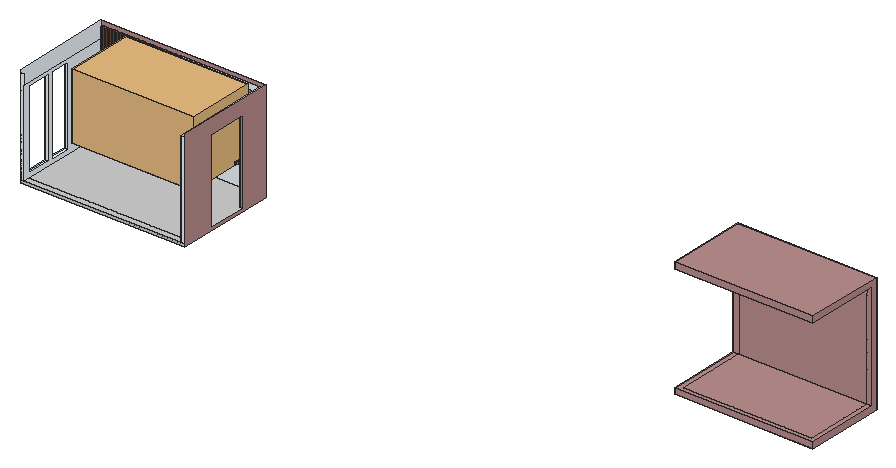
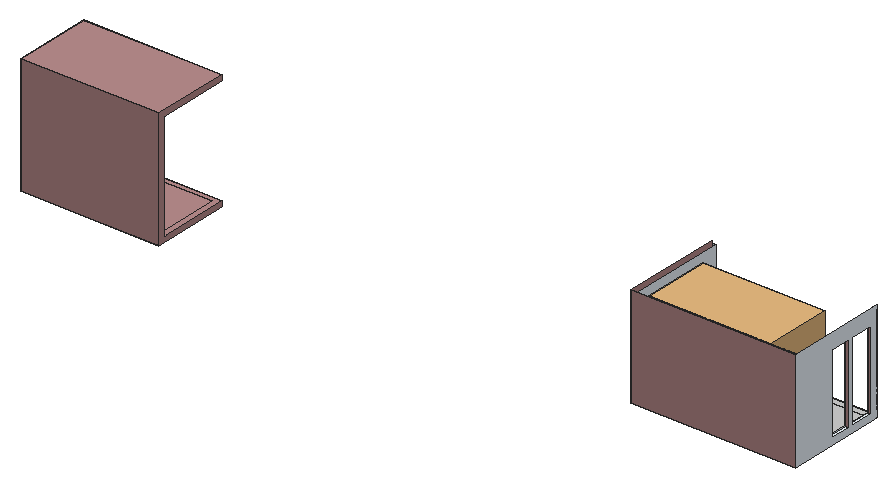
# SketchUp Ruby script. Lengths in inches.
U = 1.inch
M = Sketchup.active_model
def pt(a) = Geom::Point3d.new(a.map { |v| v * U })
def face(e, loops, mat)
  f = e.add_face(loops[0].map { |a| pt(a) })
  loops[1..].each { |l| e.add_face(l.map { |a| pt(a) }).erase! }
  f.material = f.back_material = mat if mat
  f
end
# faces: each face lists its corners as indices into pts; further lists are holes
def faces(e, pts, list, mat = nil) = list.each { |f| face(e, (f[0].is_a?(Array) ? f : [f]).map { |l| l.map { |i| pts[i] } }, mat) }
# xy, xz, yz: faces in a plane at the given z, y or x. An outline is a flat list of corners, or four numbers for a rectangle; further outlines are holes
def ring(l) = l.size == 4 ? [[l[0], l[1]], [l[2], l[1]], [l[2], l[3]], [l[0], l[3]]] : l.each_slice(2).to_a
def flat(e, list, mat, &to3) = list.each { |f| face(e, (f[0].is_a?(Array) ? f : [f]).map { |l| ring(l).map { |u, v| to3.(u, v) } }, mat) }
def xy(e, z, list, mat = nil) = flat(e, list, mat) { |x, y| [x, y, z] }
def xz(e, y, list, mat = nil) = flat(e, list, mat) { |x, z| [x, y, z] }
def yz(e, x, list, mat = nil) = flat(e, list, mat) { |y, z| [x, y, z] }
def lines(e, pts, list) = list.each { |a, b| e.add_line(pt(pts[a]), pt(pts[b])) }
# prism: a flat outline (further loops are holes) pulled along v
def prism(e, loops, v, mat = nil)
  f = face(e, loops, mat); d = Geom::Vector3d.new(v.map { |x| x * U })
  f.pushpull(f.normal.samedirection?(d) ? d.length : -d.length)
end
def box(e, o, s, mat = nil) = prism(e, [[o, [o[0] + s[0], o[1], o[2]], [o[0] + s[0], o[1] + s[1], o[2]], [o[0], o[1] + s[1], o[2]]]], [0, 0, s[2]], mat)
def at(x, y, z, deg = 0) = Geom::Transformation.translation(pt([x, y, z])) * Geom::Transformation.rotation(ORIGIN, Z_AXIS, deg.degrees)
def axes(o, x, y, z) = Geom::Transformation.new([*x, 0, *y, 0, *z, 0, *pt(o).to_a, 1])
def part(name) = M.definitions.add(name)
# library, detail: a bought-in or finely detailed component or shape, given as its bounding box
def library(name, o, s) = part(name).tap { |d| box(d.entities, o, s) }
def detail(e, o, s) = box(e.add_group.entities, o, s)
def put(e, d, t, mat = nil) = e.add_instance(d, t).tap { |i| i.material = mat if mat }
def group(e, t, mat = nil) = e.add_group.tap { |g| g.transformation = t; g.material = mat if mat }.entities
root = M.entities
M.materials.add("[0093_AliceBlue]").color = [240, 248, 255]
M.materials.add("[0095_LightBlue]").color = [173, 216, 230]
M.materials.add("[0119_RosyBrown]").color = [188, 143, 143]
M.materials.add("[Carrera Marble]").color = [207, 207, 207]
M.materials.add("[Sandstone]").color = [118, 81, 52]
c1 = library("Group\#4",[-0.5,-0.5,0],[110.4375,24.3125,2.25])
c2 = library("Group\#2",[-0.5,-0.5,0],[66.38,2.78,72.7])
c3 = library("Group\#3",[-0.5,-0.5,0],[27.47,2.78,72.7])
c4 = library("Group\#5",[-0.5,-0.5,0],[170.54,94.85,92.14])
xy(root,0,[[0,0,230.5,141.75]],"[0093_AliceBlue]")
xy(root,0,[[853.51,78.57,1047.76,189.2]],"[0119_RosyBrown]")
xy(root,3.9375,[[4.95,112.24,14.18,112.24,12.9,112.62,11.89,113.04,11.67,113.13,10.5,113.79,9.83,114.27,9.42,114.56,8.43,115.46,7.54,116.46,7.01,117.21,6.77,117.55,6.125,118.72,5.61,119.96,5.25,121.24,5.02,122.56,4.95,123.89],[14.18,112.24,14.71,112.24,14.71,135.55,11.89,135.55,11.89,113.04,12.9,112.62],[14.71,112.24,16.77,137.93],[16.77,112.24,19.59,137.93],[19.59,112.24,21.65,137.93],
  [21.65,112.24,24.47,137.93],[24.47,112.24,26.53,135.55],[26.53,112.24,29.35,137.93],[29.35,112.24,31.42,137.93],[31.42,112.24,34.23,137.93],
  [34.23,112.24,36.3,137.93],[36.3,112.24,39.11,137.93],[39.11,112.24,41.18,137.93],[41.18,112.24,43.99,137.93],[43.99,112.24,46.06,137.93],
  [46.06,112.24,48.875,137.93],[48.875,112.24,50.9375,137.93],[50.9375,112.24,53.76,137.93],[53.76,112.24,55.82,137.93],[55.82,112.24,58.64,137.93],
  [58.64,112.24,60.7,137.93],[60.7,112.24,63.52,137.93],[63.52,112.24,65.58,137.93],[65.58,112.24,68.4,137.93],[68.4,112.24,70.46,137.93],
  [70.46,112.24,73.28,137.93],[73.28,112.24,75.34,137.93],[75.34,112.24,78.16,137.93],[78.16,112.24,80.22,137.93],[80.22,112.24,83.04,137.93],
  [83.04,112.24,85.1,137.93],[85.1,112.24,87.92,137.93],[87.92,112.24,89.98,137.93],[89.98,112.24,92.8,137.93],[92.8,112.24,94.86,137.93],
  [94.86,112.24,97.68,137.93],[97.68,112.24,99.74,137.93],[99.74,112.24,102.5625,137.93],[102.5625,112.24,103.53,112.24,104.625,112.3125,104.625,135.55,102.5625,135.55],[104.625,112.3125,105.02,112.34,106.47,112.64,107.44,112.99,107.44,135.55,104.625,135.55],
  [107.44,112.99,107.875,113.14,109.2,113.83,109.51,114.05,109.51,135.55,107.44,135.55],[11.89,113.04,11.89,135.55,9.83,135.55,9.83,114.27,10.5,113.79,11.67,113.13],[109.51,114.05,110.41,114.6875,111.5,115.7,112.32,116.72,112.32,135.55,109.51,135.55],[9.83,114.27,9.83,135.55,7.01,135.55,7.01,117.21,7.54,116.46,8.43,115.46,9.42,114.56],[112.32,116.72,112.43,116.86,113.2,118.13,113.79,119.5,114.05,120.42,114.05,135.55,112.32,135.55],
  [114.05,120.42,114.19,120.93,114.39,122.375,114.39,135.55,114.05,135.55],[7.01,135.55,9.83,137.93],[9.83,135.55,11.89,137.93],[11.89,135.55,14.71,137.93],[24.47,135.55,26.53,137.93],
  [102.5625,135.55,104.625,137.93],[104.625,135.55,107.44,137.93],[107.44,135.55,109.51,137.93],[109.51,135.55,112.32,137.93],[112.32,135.55,114.05,137.93],
  [114.05,135.55,114.39,137.93]],"[0119_RosyBrown]")
xy(root,3.9375,[[4.95,0,225.375,9.26],[4.95,9.26,225.375,9.26,225.375,45.11,230.5,45.11,230.5,101.93,225.375,101.93,225.375,137.93,114.39,137.93,114.39,122.375,114.19,120.93,114.05,120.42,113.79,119.5,113.2,118.13,112.43,116.86,112.32,116.72,111.5,115.7,110.41,114.6875,109.51,114.05,109.2,113.83,107.875,113.14,107.44,112.99,106.47,112.64,105.02,112.34,104.625,112.3125,103.53,112.24,4.95,112.24]],"[Carrera Marble]")
xy(root,7.75,[[853.51,78.57,1047.76,78.57,1047.76,181.57,1040.13,181.57,1040.13,86.2,861.13,86.2,861.13,181.57,853.51,181.57],[861.13,86.2,1040.13,181.57]],"[0119_RosyBrown]")
xy(root,9.5,[[0,9.26,4.95,43.72],[0,48.29,4.95,77.05]],"[0093_AliceBlue]")
xy(root,9.5,[[0,43.72,4.95,48.29]],"[0119_RosyBrown]")
xy(root,15.0625,[[14.18,112.24,103.53,115.3]],"[0119_RosyBrown]")
xy(root,16.4375,[[14.18,112.24,103.53,115.3]],"[0119_RosyBrown]")
xy(root,30.75,[[14.18,112.24,103.53,112.24,105.02,112.34,106.47,112.64,107.875,113.14,109.2,113.83,110.41,114.6875,111.5,115.7,112.43,116.86,113.2,118.13,113.79,119.5,114.19,120.93,114.39,122.375,114.39,135.55,4.95,135.55,4.95,123.89,5.02,122.56,5.25,121.24,5.61,119.96,6.125,118.72,6.77,117.55,7.54,116.46,8.43,115.46,9.42,114.56,10.5,113.79,11.67,113.13,12.9,112.62]],"[0119_RosyBrown]")
xy(root,35.24,[[4.97,133.77,70.35,135.55],[87.92,133.77,114.39,135.55]],"[0095_LightBlue]")
xy(root,46.22,[[[137.0625,109.13,135.97,109.21,135.02,109.41,134.1,109.73,133.23,110.18,132.43,110.74,131.72,111.4,131.1,112.16,130.59,112.99,130.2,113.88,129.93,114.82,129.79,115.78,129.78,116.98,129.78,134.53,209.98,134.53,209.98,117.22,209.81,116.2,209.49,115.13,209.04,114.11,208.48,113.15,207.8,112.27,207.02,111.48,206.15,110.79,205.2,110.21,204.18,109.74,203.125,109.41,202.03,109.21,200.8125,109.13],[137.09,109.92,200.79,109.92,201.93,109.99,202.93,110.18,203.9,110.48,204.83,110.9,205.69,111.43,206.49,112.07,207.2,112.79,207.82,113.6,208.34,114.47,208.75,115.4,209.04,116.38,209.19,117.29,209.19,133.74,130.57,133.74,130.57,116.98,130.58,115.84,130.7,114.98,130.94,114.15,131.29,113.35,131.74,112.61,132.29,111.94,132.93,111.35,133.64,110.85,134.41,110.46,135.23,110.17,136.08,109.99]]],"[0119_RosyBrown]")
xy(root,47.91,[[[136.95,105.74,135.51,105.84,134.1,106.13,132.75,106.61,131.47,107.27,130.29,108.09,129.24,109.07,128.33,110.18,127.57,111.41,127,112.72,126.6,114.11,126.4,115.53,126.39,116.97,126.39,137.93,213.375,137.93,213.375,116.94,213.12,115.43,212.68,113.96,212.07,112.5625,211.3,111.25,210.36,110.04,209.29,108.95,208.1,108,206.79,107.2,205.4,106.57,203.95,106.11,202.44,105.83,200.92,105.74],[137.0625,109.13,200.8125,109.13,202.03,109.21,203.125,109.41,204.18,109.74,205.2,110.21,206.15,110.79,207.02,111.48,207.8,112.27,208.48,113.15,209.04,114.11,209.49,115.13,209.81,116.2,209.98,117.22,209.98,134.53,129.78,134.53,129.78,116.98,129.79,115.78,129.93,114.82,130.2,113.88,130.59,112.99,131.1,112.16,131.72,111.4,132.43,110.74,133.23,110.18,134.1,109.73,135.02,109.41,135.97,109.21]],[137.09,109.92,136.08,109.99,135.23,110.17,134.41,110.46,133.64,110.85,132.93,111.35,132.29,111.94,131.74,112.61,131.29,113.35,130.94,114.15,130.7,114.98,130.58,115.84,130.57,116.98,130.57,133.74,209.19,133.74,209.19,117.29,209.04,116.38,208.75,115.4,208.34,114.47,207.82,113.6,207.2,112.79,206.49,112.07,205.69,111.43,204.83,110.9,203.9,110.48,202.93,110.18,201.93,109.99,200.79,109.92]],"[0119_RosyBrown]")
xy(root,51.66,[[136.95,105.74,200.92,105.74,202.44,105.83,203.95,106.11,205.4,106.57,206.79,107.2,208.1,108,209.29,108.95,210.36,110.04,211.3,111.25,212.07,112.5625,212.68,113.96,213.12,115.43,213.375,116.94,213.375,137.93,126.39,137.93,126.39,116.97,126.4,115.53,126.6,114.11,127,112.72,127.57,111.41,128.33,110.18,129.24,109.07,130.29,108.09,131.47,107.27,132.75,106.61,134.1,106.13,135.51,105.84]],"[0119_RosyBrown]")
xy(root,107.93,[[101.15,133.77,114.39,135.55]],"[0095_LightBlue]")
xy(root,157.52,[[853.51,78.57,861.13,181.57],[861.13,78.57,1040.13,181.57],[1040.13,78.57,1047.76,181.57]],"[0119_RosyBrown]")
xy(root,166,[[853.51,78.57,1047.76,189.2]],"[0119_RosyBrown]")
xz(root,0,[[0,3.9375,4.95,138.36],[225.375,3.9375,230.5,138.36]],"[0093_AliceBlue]")
xz(root,0,[[0,0,230.5,3.9375]],"[Carrera Marble]")
xz(root,9.26,[[0,9.5,4.95,119.86]],"[0119_RosyBrown]")
xz(root,43.72,[[0,9.5,4.95,119.86]],"[0093_AliceBlue]")
xz(root,45.11,[[225.375,3.9375,230.5,121.64]],"[0119_RosyBrown]")
xz(root,48.29,[[0,9.5,4.95,119.86]],"[0119_RosyBrown]")
xz(root,77.05,[[0,9.5,4.95,119.86]],"[0093_AliceBlue]")
xz(root,78.57,[[853.51,0,1047.76,7.75],[853.51,157.52,1047.76,166]],"[0119_RosyBrown]")
xz(root,101.93,[[225.375,3.9375,230.5,121.64]],"[0119_RosyBrown]")
xz(root,105.74,[[136.95,47.91,200.92,51.66]],"[0119_RosyBrown]")
xz(root,109.13,[[137.0625,46.22,200.8125,46.6],[137.0625,46.6,200.8125,47.91]],"[0119_RosyBrown]")
xz(root,109.92,[[137.09,46.22,200.79,46.6],[137.09,46.6,200.79,47.91]],"[0119_RosyBrown]")
xz(root,112.24,[[14.18,3.9375,103.53,15.0625],[14.18,16.4375,103.53,28.5]],"[0119_RosyBrown]")
xz(root,115.3,[[14.18,15.0625,103.53,16.4375]],"[0119_RosyBrown]")
xz(root,131.99,[[4.97,35.24,70.35,35.24,70.35,92.61,70.01,94.53,69.47,96.4,68.71,98.19,67.77,99.89,66.64,101.48,65.34,102.93,63.89,104.22,62.31,105.35,60.61,106.3,58.8125,107.05,56.95,107.6,55.03,107.93,4.97,107.93],[87.92,35.24,114.39,35.24,114.39,107.93,101.15,107.93,99.43,107.82,97.73,107.48,96.09,106.93,94.54,106.16,93.1,105.2,91.8,104.06,90.66,102.76,89.69,101.32,88.93,99.76,88.37,98.125,88.03,96.43,87.92,94.7]],"[0095_LightBlue]")
xz(root,133.74,[[130.57,46.22,209.19,46.6],[130.57,46.6,209.19,47.91]],"[0119_RosyBrown]")
xz(root,134.53,[[129.78,46.22,209.98,46.6],[129.78,46.6,209.98,47.91]],"[0119_RosyBrown]")
xz(root,135.55,[[4.95,3.9375,26.53,30.75],[26.53,3.9375,114.39,30.75],[4.95,35.24,4.97,107.93],[4.97,35.24,26.53,107.93],[26.53,35.24,26.53,107.93,55.03,107.93,56.95,107.6,58.8125,107.05,60.61,106.3,62.31,105.35,63.89,104.22,65.34,102.93,66.64,101.48,67.77,99.89,68.71,98.19,69.47,96.4,70.01,94.53,70.35,92.61,70.35,35.24],
  [87.92,35.24,87.92,94.7,88.03,96.43,88.37,98.125,88.93,99.76,89.69,101.32,90.66,102.76,91.8,104.06,93.1,105.2,94.54,106.16,96.09,106.93,97.73,107.48,99.43,107.82,101.15,107.93,114.39,107.93,114.39,35.24]],"[0119_RosyBrown]")
xz(root,137.93,[[7.01,3.9375,9.83,138.36],[11.89,3.9375,14.71,138.36],[16.77,3.9375,19.59,138.36],[21.65,3.9375,24.47,138.36],[26.53,3.9375,29.35,138.36],
  [31.42,3.9375,34.23,138.36],[36.3,3.9375,39.11,138.36],[41.18,3.9375,43.99,138.36],[46.06,3.9375,48.875,138.36],[50.9375,3.9375,53.76,138.36],
  [55.82,3.9375,58.64,138.36],[60.7,3.9375,63.52,138.36],[65.58,3.9375,68.4,138.36],[70.46,3.9375,73.28,138.36],[75.34,3.9375,78.16,138.36],
  [80.22,3.9375,83.04,138.36],[85.1,3.9375,87.92,138.36],[89.98,3.9375,92.8,138.36],[94.86,3.9375,97.68,138.36],[99.74,3.9375,102.5625,138.36],
  [104.625,3.9375,107.44,138.36],[109.51,3.9375,112.32,138.36],[[114.39,3.9375,225.375,138.36],[189.375,103.42,213.375,130.36],[151.09,86.86,188.68,103.11],[151.09,115.49,188.68,130.36],[151.09,103.42,188.68,115.3],[189.375,86.86,213.375,103.11],[126.39,86.86,150.39,102.8],[126.39,115.49,150.39,130.36],[126.39,47.91,213.375,51.66],[126.39,103.42,150.39,115.3]]],"[0093_AliceBlue]")
xz(root,137.93,[[9.83,3.9375,11.89,138.36],[14.71,3.9375,16.77,138.36],[19.59,3.9375,21.65,138.36],[24.47,3.9375,26.53,138.36],[29.35,3.9375,31.42,138.36],
  [34.23,3.9375,36.3,138.36],[39.11,3.9375,41.18,138.36],[43.99,3.9375,46.06,138.36],[48.875,3.9375,50.9375,138.36],[53.76,3.9375,55.82,138.36],
  [58.64,3.9375,60.7,138.36],[63.52,3.9375,65.58,138.36],[68.4,3.9375,70.46,138.36],[73.28,3.9375,75.34,138.36],[78.16,3.9375,80.22,138.36],
  [83.04,3.9375,85.1,138.36],[87.92,3.9375,89.98,138.36],[92.8,3.9375,94.86,138.36],[97.68,3.9375,99.74,138.36],[102.5625,3.9375,104.625,138.36],
  [107.44,3.9375,109.51,138.36],[112.32,3.9375,114.05,138.36],[114.05,3.9375,114.39,138.36]],"[0119_RosyBrown]")
xz(root,141.75,[[0,0,230.5,141.75]],"[0119_RosyBrown]")
xz(root,181.57,[[853.51,7.75,861.13,157.52],[861.13,7.75,1040.13,157.52],[1040.13,7.75,1047.76,157.52]],"[0119_RosyBrown]")
xz(root,189.2,[[853.51,0,1047.76,166]],"[0119_RosyBrown]")
yz(root,0,[[[0,0,141.75,141.75],[9.26,9.5,43.72,9.5,43.72,119.86,48.29,119.86,48.29,9.5,77.05,9.5,77.05,119.86,9.26,119.86]]],"[0093_AliceBlue]")
yz(root,4.95,[[[0,3.9375,123.89,3.9375,123.89,30.75,135.55,30.75,135.55,3.9375,137.93,3.9375,137.93,138.36,135.55,138.36,135.55,123.05,0,123.05],[9.26,9.5,9.26,119.86,77.05,119.86,77.05,9.5,48.29,9.5,48.29,119.86,43.72,119.86,43.72,9.5]]],"[0093_AliceBlue]")
yz(root,4.95,[[123.89,3.9375,135.55,28.5],[123.89,28.5,135.55,30.75]],"[0119_RosyBrown]")
yz(root,4.97,[[131.99,35.24,133.77,107.93],[133.77,35.24,135.55,107.93]],"[0119_RosyBrown]")
yz(root,14.18,[[112.24,15.0625,115.3,16.4375]],"[0119_RosyBrown]")
yz(root,26.53,[[135.55,3.9375,137.93,138.36]],"[Sandstone]")
yz(root,70.35,[[133.77,35.24,135.55,92.61]],"[0095_LightBlue]")
yz(root,87.92,[[133.77,35.24,135.55,94.7]],"[0119_RosyBrown]")
yz(root,103.53,[[112.24,15.0625,115.3,16.4375]],"[0119_RosyBrown]")
yz(root,114.39,[[133.77,35.24,135.55,107.93]],"[0095_LightBlue]")
yz(root,114.39,[[122.375,3.9375,135.55,28.5]],"[0119_RosyBrown]")
yz(root,126.39,[[116.97,47.91,137.93,51.66]],"[0119_RosyBrown]")
yz(root,129.78,[[116.98,46.22,134.53,46.6],[116.98,46.6,134.53,47.91]],"[0119_RosyBrown]")
yz(root,130.57,[[116.98,46.22,133.74,46.6],[116.98,46.6,133.74,47.91]],"[0119_RosyBrown]")
yz(root,209.19,[[117.29,46.22,133.74,46.6],[117.29,46.6,133.74,47.91]],"[0119_RosyBrown]")
yz(root,209.98,[[117.22,46.22,134.53,46.6],[117.22,46.6,134.53,47.91]],"[0119_RosyBrown]")
yz(root,213.375,[[116.94,47.91,137.93,51.66]],"[0119_RosyBrown]")
yz(root,225.375,[[0,3.9375,0,138.36,137.93,138.36,137.93,3.9375,101.93,3.9375,101.93,121.64,45.11,121.64,45.11,3.9375]],"[0093_AliceBlue]")
yz(root,230.5,[[[0,0,141.75,141.75],[45.11,3.9375,101.93,121.64]]],"[0119_RosyBrown]")
yz(root,853.51,[[78.57,0,78.57,7.75,181.57,7.75,181.57,157.52,78.57,157.52,78.57,166,189.2,166,189.2,0]],"[0119_RosyBrown]")
yz(root,1047.76,[[78.57,0,189.2,0,189.2,166,78.57,166,78.57,157.52,181.57,157.52,181.57,7.75,78.57,7.75]],"[0119_RosyBrown]")
p = [[14.18,112.24,16.4375],[14.18,112.24,28.5],[12.9,112.62,28.5],[12.9,112.62,3.9375],[14.18,112.24,3.9375],[14.18,112.24,15.0625],
  [105.02,112.34,3.9375],[105.02,112.34,28.5],[103.53,112.24,28.5],[103.53,112.24,16.4375],[103.53,112.24,15.0625],[103.53,112.24,3.9375],
  [104.625,112.3125,3.9375],[106.47,112.64,3.9375],[106.47,112.64,28.5],[11.67,113.13,28.5],[11.67,113.13,3.9375],[11.89,113.04,3.9375],
  [107.875,113.14,3.9375],[107.875,113.14,28.5],[107.44,112.99,3.9375],[10.5,113.79,28.5],[10.5,113.79,3.9375],[109.2,113.83,3.9375],
  [109.2,113.83,28.5],[9.42,114.56,28.5],[9.42,114.56,3.9375],[9.83,114.27,3.9375],[110.41,114.6875,3.9375],[110.41,114.6875,28.5],
  [109.51,114.05,3.9375],[8.43,115.46,28.5],[8.43,115.46,3.9375],[111.5,115.7,3.9375],[111.5,115.7,28.5],[7.54,116.46,28.5],
  [7.54,116.46,3.9375],[112.43,116.86,3.9375],[112.43,116.86,28.5],[112.32,116.72,3.9375],[6.77,117.55,28.5],[6.77,117.55,3.9375],
  [7.01,117.21,3.9375],[113.2,118.13,3.9375],[113.2,118.13,28.5],[6.125,118.72,28.5],[6.125,118.72,3.9375],[113.79,119.5,3.9375],
  [113.79,119.5,28.5],[5.61,119.96,28.5],[5.61,119.96,3.9375],[114.19,120.93,3.9375],[114.19,120.93,28.5],[114.05,120.42,3.9375],
  [5.25,121.24,28.5],[5.25,121.24,3.9375],[114.39,122.375,3.9375],[114.39,122.375,28.5],[5.02,122.56,28.5],[5.02,122.56,3.9375],
  [4.95,123.89,28.5],[4.95,123.89,3.9375],[137.0625,109.13,46.22],[137.0625,109.13,46.6],[135.97,109.21,46.6],[135.97,109.21,46.22],
  [202.03,109.21,46.22],[202.03,109.21,46.6],[200.8125,109.13,46.6],[200.8125,109.13,46.22],[135.02,109.41,46.6],[135.02,109.41,46.22],
  [203.125,109.41,46.22],[203.125,109.41,46.6],[134.1,109.73,46.6],[134.1,109.73,46.22],[204.18,109.74,46.22],[204.18,109.74,46.6],
  [133.23,110.18,46.6],[133.23,110.18,46.22],[205.2,110.21,46.22],[205.2,110.21,46.6],[136.08,109.99,46.22],[136.08,109.99,46.6],
  [137.09,109.92,46.6],[137.09,109.92,46.22],[200.79,109.92,46.22],[200.79,109.92,46.6],[201.93,109.99,46.6],[201.93,109.99,46.22],
  [135.23,110.17,46.22],[135.23,110.17,46.6],[202.93,110.18,46.6],[202.93,110.18,46.22],[132.43,110.74,46.6],[132.43,110.74,46.22],
  [134.41,110.46,46.22],[134.41,110.46,46.6],[203.9,110.48,46.6],[203.9,110.48,46.22],[206.15,110.79,46.22],[206.15,110.79,46.6],
  [133.64,110.85,46.22],[133.64,110.85,46.6],[204.83,110.9,46.6],[204.83,110.9,46.22],[131.72,111.4,46.6],[131.72,111.4,46.22],
  [207.02,111.48,46.22],[207.02,111.48,46.6],[132.93,111.35,46.22],[132.93,111.35,46.6],[205.69,111.43,46.6],[205.69,111.43,46.22],
  [131.1,112.16,46.6],[131.1,112.16,46.22],[132.29,111.94,46.22],[132.29,111.94,46.6],[206.49,112.07,46.6],[206.49,112.07,46.22],
  [207.8,112.27,46.22],[207.8,112.27,46.6],[131.74,112.61,46.22],[131.74,112.61,46.6],[207.2,112.79,46.6],[207.2,112.79,46.22],
  [130.59,112.99,46.6],[130.59,112.99,46.22],[208.48,113.15,46.22],[208.48,113.15,46.6],[131.29,113.35,46.22],[131.29,113.35,46.6],
  [207.82,113.6,46.6],[207.82,113.6,46.22],[130.2,113.88,46.6],[130.2,113.88,46.22],[209.04,114.11,46.22],[209.04,114.11,46.6],
  [130.94,114.15,46.22],[130.94,114.15,46.6],[208.34,114.47,46.6],[208.34,114.47,46.22],[129.93,114.82,46.6],[129.93,114.82,46.22],
  [130.7,114.98,46.22],[130.7,114.98,46.6],[209.49,115.13,46.22],[209.49,115.13,46.6],[208.75,115.4,46.6],[208.75,115.4,46.22],
  [129.79,115.78,46.6],[129.79,115.78,46.22],[130.58,115.84,46.22],[130.58,115.84,46.6],[209.81,116.2,46.22],[209.81,116.2,46.6],
  [209.04,116.38,46.6],[209.04,116.38,46.22],[129.78,116.98,46.6],[129.78,116.98,46.22],[130.57,116.98,46.22],[130.57,116.98,46.6],
  [209.98,117.22,46.22],[209.98,117.22,46.6],[209.19,117.29,46.6],[209.19,117.29,46.22],[135.97,109.21,47.91],[137.0625,109.13,47.91],
  [200.8125,109.13,47.91],[202.03,109.21,47.91],[135.02,109.41,47.91],[203.125,109.41,47.91],[134.1,109.73,47.91],[204.18,109.74,47.91],
  [133.23,110.18,47.91],[205.2,110.21,47.91],[137.09,109.92,47.91],[136.08,109.99,47.91],[201.93,109.99,47.91],[200.79,109.92,47.91],
  [135.23,110.17,47.91],[202.93,110.18,47.91],[132.43,110.74,47.91],[134.41,110.46,47.91],[203.9,110.48,47.91],[206.15,110.79,47.91],
  [133.64,110.85,47.91],[204.83,110.9,47.91],[131.72,111.4,47.91],[207.02,111.48,47.91],[132.93,111.35,47.91],[205.69,111.43,47.91],
  [131.1,112.16,47.91],[132.29,111.94,47.91],[206.49,112.07,47.91],[207.8,112.27,47.91],[131.74,112.61,47.91],[207.2,112.79,47.91],
  [130.59,112.99,47.91],[208.48,113.15,47.91],[131.29,113.35,47.91],[207.82,113.6,47.91],[130.2,113.88,47.91],[209.04,114.11,47.91],
  [130.94,114.15,47.91],[208.34,114.47,47.91],[129.93,114.82,47.91],[130.7,114.98,47.91],[209.49,115.13,47.91],[208.75,115.4,47.91],
  [129.79,115.78,47.91],[130.58,115.84,47.91],[209.81,116.2,47.91],[209.04,116.38,47.91],[129.78,116.98,47.91],[130.57,116.98,47.91],
  [209.98,117.22,47.91],[209.19,117.29,47.91],[136.95,105.74,51.66],[135.51,105.84,51.66],[135.51,105.84,47.91],[136.95,105.74,47.91],
  [202.44,105.83,51.66],[200.92,105.74,51.66],[200.92,105.74,47.91],[202.44,105.83,47.91],[134.1,106.13,51.66],[134.1,106.13,47.91],
  [203.95,106.11,51.66],[203.95,106.11,47.91],[132.75,106.61,51.66],[132.75,106.61,47.91],[205.4,106.57,51.66],[205.4,106.57,47.91],
  [131.47,107.27,51.66],[131.47,107.27,47.91],[206.79,107.2,51.66],[206.79,107.2,47.91],[208.1,108,51.66],[208.1,108,47.91],
  [130.29,108.09,51.66],[130.29,108.09,47.91],[209.29,108.95,51.66],[209.29,108.95,47.91],[129.24,109.07,51.66],[129.24,109.07,47.91],
  [210.36,110.04,51.66],[210.36,110.04,47.91],[128.33,110.18,51.66],[128.33,110.18,47.91],[211.3,111.25,51.66],[211.3,111.25,47.91],
  [127.57,111.41,51.66],[127.57,111.41,47.91],[212.07,112.5625,51.66],[212.07,112.5625,47.91],[127,112.72,51.66],[127,112.72,47.91],
  [212.68,113.96,51.66],[212.68,113.96,47.91],[126.6,114.11,51.66],[126.6,114.11,47.91],[213.12,115.43,51.66],[213.12,115.43,47.91],
  [126.4,115.53,51.66],[126.4,115.53,47.91],[213.375,116.94,51.66],[213.375,116.94,47.91],[126.39,116.97,51.66],[126.39,116.97,47.91],
  [87.92,135.55,94.7],[87.92,133.77,94.7],[88.03,133.77,96.43],[88.03,135.55,96.43],[88.37,133.77,98.125],[88.37,135.55,98.125],
  [88.93,133.77,99.76],[88.93,135.55,99.76],[89.69,133.77,101.32],[89.69,135.55,101.32],[90.66,133.77,102.76],[90.66,135.55,102.76],
  [91.8,133.77,104.06],[91.8,135.55,104.06],[93.1,133.77,105.2],[93.1,135.55,105.2],[94.54,133.77,106.16],[94.54,135.55,106.16],
  [96.09,133.77,106.93],[96.09,135.55,106.93],[97.73,133.77,107.48],[97.73,135.55,107.48],[99.43,133.77,107.82],[99.43,135.55,107.82],
  [101.15,133.77,107.93],[101.15,135.55,107.93]]
faces(root,p,[[0,1,2,3,4,5],[6,7,8,9,10,11,12],[13,14,7,6],[3,2,15,16,17],[18,19,14,13,20],[16,15,21,22],[23,24,19,18],[22,21,25,26,27],
  [28,29,24,23,30],[26,25,31,32],[33,34,29,28],[32,31,35,36],[37,38,34,33,39],[36,35,40,41,42],[43,44,38,37],[41,40,45,46],
  [47,48,44,43],[46,45,49,50],[51,52,48,47,53],[50,49,54,55],[56,57,52,51],[55,54,58,59],[59,58,60,61],[62,63,64,65],
  [66,67,68,69],[65,64,70,71],[72,73,67,66],[71,70,74,75],[76,77,73,72],[75,74,78,79],[80,81,77,76],[82,83,84,85],
  [86,87,88,89],[90,91,83,82],[89,88,92,93],[79,78,94,95],[96,97,91,90],[93,92,98,99],[100,101,81,80],[102,103,97,96],
  [99,98,104,105],[95,94,106,107],[108,109,101,100],[110,111,103,102],[105,104,112,113],[107,106,114,115],[116,117,111,110],[113,112,118,119],
  [120,121,109,108],[122,123,117,116],[119,118,124,125],[115,114,126,127],[128,129,121,120],[130,131,123,122],[125,124,132,133],[127,126,134,135],
  [136,137,129,128],[138,139,131,130],[133,132,140,141],[135,134,142,143],[144,145,139,138],[146,147,137,136],[141,140,148,149],[143,142,150,151],
  [152,153,145,144],[154,155,147,146],[149,148,156,157],[151,150,158,159],[160,161,153,152],[162,163,155,154],[157,156,164,165],[166,64,63,167],
  [168,68,67,169],[170,70,64,166],[169,67,73,171],[172,74,70,170],[171,73,77,173],[174,78,74,172],[173,77,81,175],[176,84,83,177],
  [178,88,87,179],[177,83,91,180],[181,92,88,178],[182,94,78,174],[180,91,97,183],[184,98,92,181],[175,81,101,185],[183,97,103,186],
  [187,104,98,184],[188,106,94,182],[185,101,109,189],[186,103,111,190],[191,112,104,187],[192,114,106,188],[190,111,117,193],[194,118,112,191],
  [189,109,121,195],[193,117,123,196],[197,124,118,194],[198,126,114,192],[195,121,129,199],[196,123,131,200],[201,132,124,197],[202,134,126,198],
  [199,129,137,203],[200,131,139,204],[205,140,132,201],[206,142,134,202],[204,139,145,207],[203,137,147,208],[209,148,140,205],[210,150,142,206],
  [207,145,153,211],[208,147,155,212],[213,156,148,209],[214,158,150,210],[211,153,161,215],[212,155,163,216],[217,164,156,213],[218,219,220,221],
  [222,223,224,225],[219,226,227,220],[228,222,225,229],[226,230,231,227],[232,228,229,233],[230,234,235,231],[236,232,233,237],[238,236,237,239],
  [234,240,241,235],[242,238,239,243],[240,244,245,241],[246,242,243,247],[244,248,249,245],[250,246,247,251],[248,252,253,249],[254,250,251,255],
  [252,256,257,253],[258,254,255,259],[256,260,261,257],[262,258,259,263],[260,264,265,261],[266,262,263,267],[264,268,269,265]],"[0119_RosyBrown]")
faces(root,p,[[270,271,272,273],[273,272,274,275],[275,274,276,277],[277,276,278,279],[279,278,280,281],[281,280,282,283],[283,282,284,285],[285,284,286,287],
  [287,286,288,289],[289,288,290,291],[291,290,292,293],[293,292,294,295]],"[0095_LightBlue]")
g1 = group(root,at(4.95,135.55,3.9375),"[0119_RosyBrown]")
xz(g1,0,[[0,0,2.0625,134.42],[4.88,0,6.94,134.42],[9.76,0,11.82,134.42],[14.64,0,16.7,134.42],[19.52,0,21.59,134.42],
  [24.4,0,26.47,134.42],[29.28,0,31.35,134.42],[34.16,0,36.23,134.42],[39.05,0,41.11,134.42],[43.93,0,45.99,134.42],
  [48.81,0,50.87,134.42],[53.6875,0,55.75,134.42],[58.57,0,60.63,134.42],[63.45,0,65.51,134.42],[68.33,0,70.39,134.42],
  [73.21,0,75.27,134.42],[78.09,0,80.15,134.42],[82.97,0,85.03,134.42],[87.85,0,89.91,134.42],[92.73,0,94.8,134.42],
  [97.61,0,99.68,134.42],[102.49,0,104.56,134.42],[107.375,0,109.4375,134.42]],"[Sandstone]")
yz(g1,0,[[0,0,2.375,134.42]],"[Sandstone]")
yz(g1,2.0625,[[0,0,2.375,134.42]],"[Sandstone]")
yz(g1,4.88,[[0,0,2.375,134.42]])
yz(g1,6.94,[[0,0,2.375,134.42]],"[Sandstone]")
yz(g1,9.76,[[0,0,2.375,134.42]])
yz(g1,11.82,[[0,0,2.375,134.42]],"[Sandstone]")
yz(g1,14.64,[[0,0,2.375,134.42]])
yz(g1,16.7,[[0,0,2.375,134.42]],"[Sandstone]")
yz(g1,19.52,[[0,0,2.375,134.42]])
yz(g1,24.4,[[0,0,2.375,134.42]])
yz(g1,26.47,[[0,0,2.375,134.42]],"[Sandstone]")
yz(g1,29.28,[[0,0,2.375,134.42]])
yz(g1,31.35,[[0,0,2.375,134.42]],"[Sandstone]")
yz(g1,34.16,[[0,0,2.375,134.42]])
yz(g1,36.23,[[0,0,2.375,134.42]],"[Sandstone]")
yz(g1,39.05,[[0,0,2.375,134.42]])
yz(g1,41.11,[[0,0,2.375,134.42]],"[Sandstone]")
yz(g1,43.93,[[0,0,2.375,134.42]])
yz(g1,45.99,[[0,0,2.375,134.42]],"[Sandstone]")
yz(g1,48.81,[[0,0,2.375,134.42]])
yz(g1,50.87,[[0,0,2.375,134.42]],"[Sandstone]")
yz(g1,53.6875,[[0,0,2.375,134.42]])
yz(g1,55.75,[[0,0,2.375,134.42]],"[Sandstone]")
yz(g1,58.57,[[0,0,2.375,134.42]])
yz(g1,60.63,[[0,0,2.375,134.42]],"[Sandstone]")
yz(g1,63.45,[[0,0,2.375,134.42]])
yz(g1,65.51,[[0,0,2.375,134.42]],"[Sandstone]")
yz(g1,68.33,[[0,0,2.375,134.42]])
yz(g1,70.39,[[0,0,2.375,134.42]],"[Sandstone]")
yz(g1,73.21,[[0,0,2.375,134.42]])
yz(g1,75.27,[[0,0,2.375,134.42]],"[Sandstone]")
yz(g1,78.09,[[0,0,2.375,134.42]])
yz(g1,80.15,[[0,0,2.375,134.42]],"[Sandstone]")
yz(g1,82.97,[[0,0,2.375,134.42]])
yz(g1,85.03,[[0,0,2.375,134.42]],"[Sandstone]")
yz(g1,87.85,[[0,0,2.375,134.42]])
yz(g1,89.91,[[0,0,2.375,134.42]],"[Sandstone]")
yz(g1,92.73,[[0,0,2.375,134.42]])
yz(g1,94.8,[[0,0,2.375,134.42]],"[Sandstone]")
yz(g1,97.61,[[0,0,2.375,134.42]])
yz(g1,99.68,[[0,0,2.375,134.42]],"[Sandstone]")
yz(g1,102.49,[[0,0,2.375,134.42]])
yz(g1,104.56,[[0,0,2.375,134.42]],"[Sandstone]")
yz(g1,107.375,[[0,0,2.375,134.42]])
yz(g1,109.4375,[[0,0,2.375,134.42]],"[Sandstone]")
put(root,c1,at(4.95,112.24,28.5),"[0119_RosyBrown]")
put(root,c2,at(4.97,131.99,35.24),"[0095_LightBlue]")
put(root,c3,at(87.92,131.99,35.24),"[0095_LightBlue]")
put(root,c4,at(40.44,40.68,46.6),"[0119_RosyBrown]")
